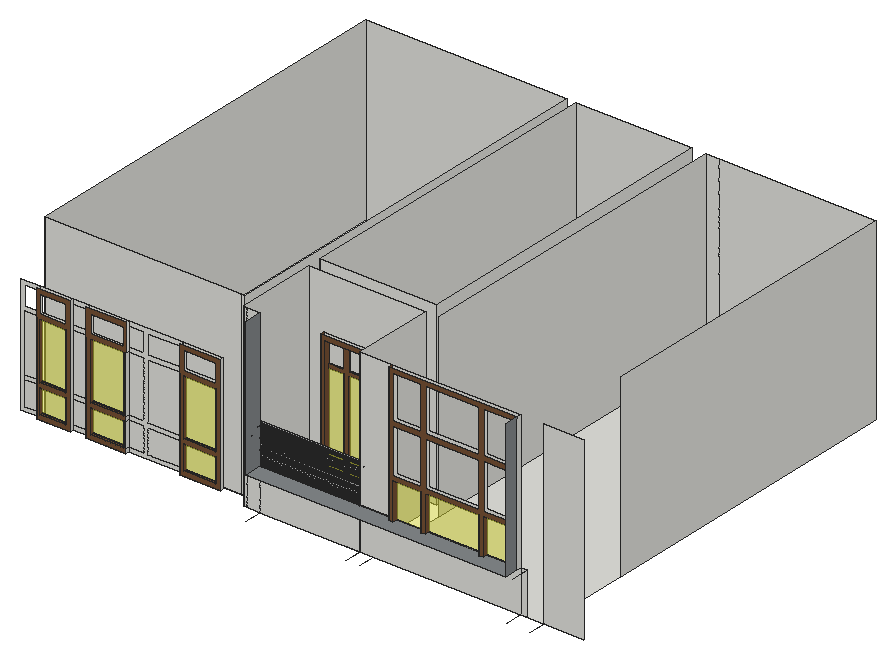
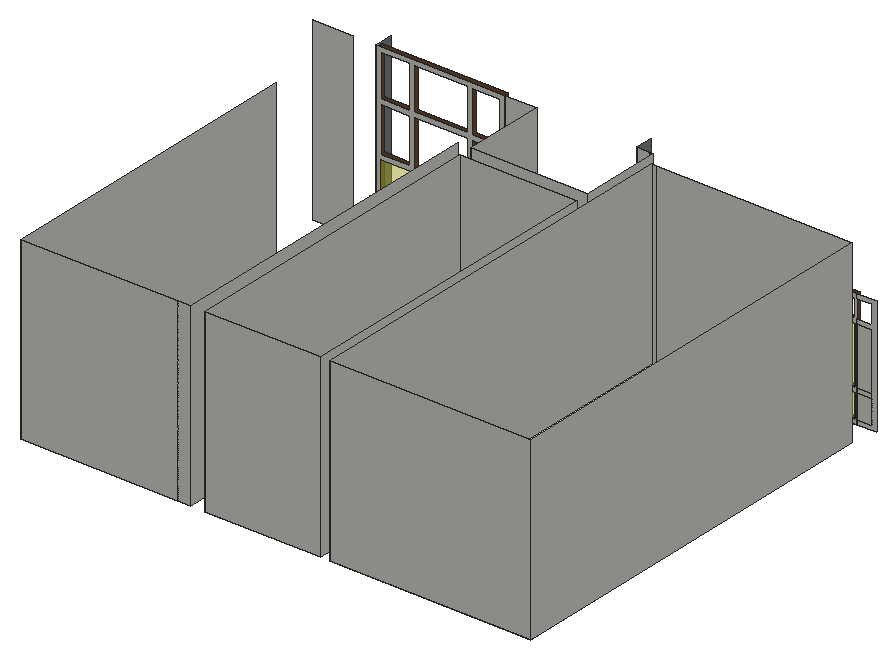
# SketchUp Ruby script. Lengths in inches.
U = 1.inch
M = Sketchup.active_model
def pt(a) = Geom::Point3d.new(a.map { |v| v * U })
def face(e, loops, mat)
  f = e.add_face(loops[0].map { |a| pt(a) })
  loops[1..].each { |l| e.add_face(l.map { |a| pt(a) }).erase! }
  f.material = f.back_material = mat if mat
  f
end
# faces: each face lists its corners as indices into pts; further lists are holes
def faces(e, pts, list, mat = nil) = list.each { |f| face(e, (f[0].is_a?(Array) ? f : [f]).map { |l| l.map { |i| pts[i] } }, mat) }
# xy, xz, yz: faces in a plane at the given z, y or x. An outline is a flat list of corners, or four numbers for a rectangle; further outlines are holes
def ring(l) = l.size == 4 ? [[l[0], l[1]], [l[2], l[1]], [l[2], l[3]], [l[0], l[3]]] : l.each_slice(2).to_a
def flat(e, list, mat, &to3) = list.each { |f| face(e, (f[0].is_a?(Array) ? f : [f]).map { |l| ring(l).map { |u, v| to3.(u, v) } }, mat) }
def xy(e, z, list, mat = nil) = flat(e, list, mat) { |x, y| [x, y, z] }
def xz(e, y, list, mat = nil) = flat(e, list, mat) { |x, z| [x, y, z] }
def yz(e, x, list, mat = nil) = flat(e, list, mat) { |y, z| [x, y, z] }
def lines(e, pts, list) = list.each { |a, b| e.add_line(pt(pts[a]), pt(pts[b])) }
# prism: a flat outline (further loops are holes) pulled along v
def prism(e, loops, v, mat = nil)
  f = face(e, loops, mat); d = Geom::Vector3d.new(v.map { |x| x * U })
  f.pushpull(f.normal.samedirection?(d) ? d.length : -d.length)
end
def box(e, o, s, mat = nil) = prism(e, [[o, [o[0] + s[0], o[1], o[2]], [o[0] + s[0], o[1] + s[1], o[2]], [o[0], o[1] + s[1], o[2]]]], [0, 0, s[2]], mat)
def at(x, y, z, deg = 0) = Geom::Transformation.translation(pt([x, y, z])) * Geom::Transformation.rotation(ORIGIN, Z_AXIS, deg.degrees)
def axes(o, x, y, z) = Geom::Transformation.new([*x, 0, *y, 0, *z, 0, *pt(o).to_a, 1])
def part(name) = M.definitions.add(name)
# library, detail: a bought-in or finely detailed component or shape, given as its bounding box
def library(name, o, s) = part(name).tap { |d| box(d.entities, o, s) }
def detail(e, o, s) = box(e.add_group.entities, o, s)
def put(e, d, t, mat = nil) = e.add_instance(d, t).tap { |i| i.material = mat if mat }
def group(e, t, mat = nil) = e.add_group.tap { |g| g.transformation = t; g.material = mat if mat }.entities
root = M.entities
M.materials.add("[0132_LightGray]").color = [169, 169, 169]
M.materials.add("[Blacktop Old 01]").color = [132, 136, 139]
M.materials.add("[Sandstone]").color = [118, 81, 52]
M.materials.add("[Translucent Glass Blue]").color = [254, 255, 58]
M.materials["[Translucent Glass Blue]"].alpha = 0.5
xy(root,123,[[149.5625,107.5,227.6875,116.5],[236.6875,107.5,351,385.8125],[9,116.5,143.5625,385.8125],[149.5625,116.5,227.6875,116.5,227.6875,162.625,219.46,162.625,219.46,159.625,216.46,159.625,216.46,162.625,208.9,162.625,208.9,161.625,205.9,161.625,205.9,162.625,198.65,162.625,198.65,161.625,195.65,161.625,195.65,162.625,176.59,162.625,176.59,161.625,173.59,161.625,173.59,162.625,162.46,162.625,162.46,159.625,159.46,159.625,159.46,162.625,149.5625,162.625],[173.59,161.625,176.59,162.625],
  [195.65,161.625,198.65,162.625],[205.9,161.625,208.9,162.625],[149.5625,171.625,227.6875,385.8125]])
xy(root,128.33,[[108.79,105.5,135.89,107.5]])
xy(root,128.33,[[12.9375,105.5,35.3125,107.5],[45.625,105.5,72.45,107.5]],"[Sandstone]")
xy(root,131.33,[[14.63,105.5,32.375,107.5],[48.83,105.5,70.95,107.5],[111.24,105.5,132.89,107.5]],"[Sandstone]")
xy(root,147.46,[[14.63,105.5,32.375,107.5],[48.83,105.5,70.95,107.5],[111.24,105.5,132.89,107.5]],"[Sandstone]")
xy(root,150.46,[[14.63,105.5,32.375,107.5],[48.83,105.5,70.95,107.5],[111.24,105.5,132.89,107.5]],"[Sandstone]")
xy(root,150.99,[[249.13,104.5,252.13,107.5],[270.95,104.5,273.95,107.5],[309.9,104.5,312.9,107.5],[332.27,104.5,335.27,107.5]])
xy(root,150.99,[[160.6875,95.5,335.27,95.5,335.27,104.5,332.27,104.5,332.27,107.5,312.9,107.5,312.9,104.5,309.9,104.5,309.9,107.5,273.95,107.5,273.95,104.5,270.95,104.5,270.95,107.5,252.13,107.5,252.13,104.5,249.13,104.5,249.13,107.5,160.6875,107.5]],"[Blacktop Old 01]")
xz(root,104.5,[[[249.13,150.99,252.13,150.99,252.13,175.36,270.95,175.36,270.95,150.99,273.95,150.99,273.95,175.36,309.9,175.36,309.9,150.99,312.9,150.99,312.9,175.36,332.27,175.36,332.27,150.99,335.27,150.99,335.27,243,249.13,243],[273.95,178.36,309.9,208.5625],[273.95,211.5625,309.9,240],[312.9,178.36,332.27,208.5625],[252.13,178.36,270.95,208.5625],[312.9,211.5625,332.27,240],[252.13,211.5625,270.95,240]]],"[Sandstone]")
xz(root,105.5,[[[12.9375,128.33,35.3125,207.1],[14.63,150.46,32.375,188.6],[14.63,131.33,32.375,147.46],[14.63,191.6,32.375,204.1]],[[45.625,128.33,72.45,207.1],[48.83,150.46,70.95,188.6],[48.83,131.33,70.95,147.46],[48.83,191.6,70.95,204.1]],[[108.79,128.33,135.89,207.1],[111.24,150.46,132.89,188.6],[111.24,131.33,132.89,147.46],[111.24,191.6,132.89,204.1]]],"[Sandstone]")
xz(root,107.5,[[149.5625,123,151.6875,243],[151.6875,123,160.6875,243],[160.6875,123,227.6875,150.99],[227.6875,123,335.27,150.99],[335.27,123,339.25,150.99],
  [351,123,377.5,243],[0,128.33,0,207.1,12.9375,207.1,12.9375,204.1,3,204.1,3,191.6,12.9375,191.6,12.9375,188.6,3,188.6,3,131.33,12.9375,131.33,12.9375,128.33],[[12.9375,128.33,35.3125,207.1],[14.63,150.46,32.375,188.6],[14.63,131.33,32.375,147.46],[14.63,191.6,32.375,204.1]],[35.3125,128.33,35.3125,207.1,45.625,207.1,45.625,204.1,35.375,204.1,35.375,191.6,45.625,191.6,45.625,188.6,35.375,188.6,35.375,150.46,45.625,150.46,45.625,147.46,35.375,147.46,35.375,131.33,45.625,131.33,45.625,128.33],[[45.625,128.33,72.45,207.1],[48.83,150.46,70.95,188.6],[48.83,131.33,70.95,147.46],[48.83,191.6,70.95,204.1]],
  [72.45,128.33,72.45,131.33,82.75,131.33,82.75,147.46,72.45,147.46,72.45,150.46,82.75,150.46,82.75,188.6,72.45,188.6,72.45,191.6,82.75,191.6,82.75,204.1,72.45,204.1,72.45,207.1,108.79,207.1,108.79,204.1,85.75,204.1,85.75,191.6,108.79,191.6,108.79,188.6,85.75,188.6,85.75,150.46,108.79,150.46,108.79,147.46,85.75,147.46,85.75,131.33,108.79,131.33,108.79,128.33],[[108.79,128.33,135.89,207.1],[111.24,150.46,132.89,188.6],[111.24,131.33,132.89,147.46],[111.24,191.6,132.89,204.1]],[3,131.33,12.9375,147.46],[35.375,131.33,45.625,147.46],[72.45,131.33,82.75,147.46],
  [85.75,131.33,108.79,147.46],[3,147.46,12.9375,150.46],[3,150.46,12.9375,188.6],[35.375,150.46,45.625,188.6],[72.45,150.46,82.75,188.6],
  [85.75,150.46,108.79,188.6],[227.6875,150.99,249.13,243],[[249.13,150.99,249.13,243,335.27,243,335.27,150.99,332.27,150.99,332.27,175.36,312.9,175.36,312.9,150.99,309.9,150.99,309.9,175.36,273.95,175.36,273.95,150.99,270.95,150.99,270.95,175.36,252.13,175.36,252.13,150.99],[273.95,178.36,309.9,208.5625],[273.95,211.5625,309.9,240],[312.9,178.36,332.27,208.5625],[252.13,178.36,270.95,208.5625],[312.9,211.5625,332.27,240],[252.13,211.5625,270.95,240]]])
xz(root,107.5,[[14.63,131.33,32.375,147.46],[48.83,131.33,70.95,147.46],[111.24,131.33,132.89,147.46],[14.63,150.46,32.375,188.6],[48.83,150.46,70.95,188.6],
  [111.24,150.46,132.89,188.6],[252.13,150.99,270.95,175.36],[273.95,150.99,309.9,175.36],[312.9,150.99,332.27,175.36]],"[Translucent Glass Blue]")
xz(root,116.5,[[9,123,140.5625,243],[140.5625,123,143.5625,243]])
xz(root,159.625,[[159.46,123,162.46,123,162.46,204,216.46,204,216.46,123,219.46,123,219.46,207,159.46,207]],"[Sandstone]")
xz(root,161.625,[[173.59,123,176.59,123,176.59,186.83,195.65,186.83,195.65,123,198.65,123,198.65,186.83,205.9,186.83,205.9,123,208.9,123,208.9,186.83,216.46,186.83,216.46,189.41,208.9,189.41,208.9,204,205.9,204,205.9,189.41,198.65,189.41,198.65,204,195.65,204,195.65,189.41,176.59,189.41,176.59,204,173.59,204,173.59,189.41,162.46,189.41,162.46,186.83,173.59,186.83]],"[Sandstone]")
xz(root,162.625,[[149.5625,123,159.46,123,159.46,207,219.46,207,219.46,123,227.6875,123,227.6875,243,149.5625,243],[173.59,123,173.59,186.83,162.46,186.83,162.46,189.41,173.59,189.41,173.59,204,176.59,204,176.59,189.41,195.65,189.41,195.65,204,198.65,204,198.65,189.41,205.9,189.41,205.9,204,208.9,204,208.9,189.41,216.46,189.41,216.46,186.83,208.9,186.83,208.9,123,205.9,123,205.9,186.83,198.65,186.83,198.65,123,195.65,123,195.65,186.83,176.59,186.83,176.59,123]])
xz(root,162.625,[[162.46,123,173.59,186.83],[176.59,123,195.65,186.83],[198.65,123,205.9,186.83],[208.9,123,216.46,186.83]],"[Translucent Glass Blue]")
xz(root,171.625,[[149.5625,123,227.6875,243]])
xz(root,385.8125,[[9,123,143.5625,243],[149.5625,123,227.6875,243],[236.6875,123,245.6875,243],[245.6875,123,351,243]])
yz(root,9,[[116.5,123,385.8125,243]])
yz(root,12.9375,[[105.5,128.33,107.5,131.33],[105.5,131.33,107.5,147.46],[105.5,147.46,107.5,150.46],[105.5,150.46,107.5,188.6]])
yz(root,14.63,[[105.5,131.33,107.5,147.46],[105.5,150.46,107.5,188.6]],"[Sandstone]")
yz(root,32.375,[[105.5,131.33,107.5,147.46],[105.5,150.46,107.5,188.6]],"[Sandstone]")
yz(root,35.3125,[[105.5,128.33,107.5,207.1]])
yz(root,45.625,[[105.5,128.33,107.5,131.33],[105.5,131.33,107.5,147.46],[105.5,147.46,107.5,150.46],[105.5,150.46,107.5,188.6]])
yz(root,48.83,[[105.5,131.33,107.5,147.46],[105.5,150.46,107.5,188.6]],"[Sandstone]")
yz(root,70.95,[[105.5,131.33,107.5,147.46],[105.5,150.46,107.5,188.6]],"[Sandstone]")
yz(root,72.45,[[105.5,128.33,107.5,131.33],[105.5,131.33,107.5,147.46],[105.5,147.46,107.5,150.46],[105.5,150.46,107.5,188.6]])
yz(root,108.79,[[105.5,128.33,107.5,131.33],[105.5,131.33,107.5,147.46],[105.5,147.46,107.5,150.46],[105.5,150.46,107.5,188.6]])
yz(root,111.24,[[105.5,131.33,107.5,147.46],[105.5,150.46,107.5,188.6]],"[Sandstone]")
yz(root,132.89,[[105.5,131.33,107.5,147.46],[105.5,150.46,107.5,188.6]],"[Sandstone]")
yz(root,135.89,[[105.5,128.33,107.5,207.1]])
yz(root,143.5625,[[116.5,123,385.8125,243]])
yz(root,149.5625,[[[107.5,123,162.625,243],[111.46,136.84,110.83,136.92,110.24,137.16,109.74,137.55,109.35,138.06,109.11,138.64,109.02,139.27,109.11,139.91,109.35,140.49,109.74,141,110.24,141.39,110.83,141.63,111.46,141.71,112.09,141.63,112.68,141.39,113.18,141,113.57,140.49,113.8125,139.91,113.9,139.27,113.8125,138.64,113.57,138.06,113.18,137.55,112.68,137.16,112.09,136.92],[111.46,143.96,110.83,144.04,110.24,144.29,109.74,144.68,109.35,145.18,109.11,145.77,109.02,146.4,109.11,147.03,109.35,147.62,109.74,148.12,110.24,148.51,110.83,148.75,111.46,148.84,112.09,148.75,112.68,148.51,113.18,148.12,113.57,147.62,113.8125,147.03,113.9,146.4,113.8125,145.77,113.57,145.18,113.18,144.68,112.68,144.29,112.09,144.04],[111.46,151.09,110.83,151.17,110.24,151.41,109.74,151.8,109.35,152.31,109.11,152.89,109.02,153.52,109.11,154.16,109.35,154.74,109.74,155.25,110.24,155.64,110.83,155.88,111.46,155.96,112.09,155.88,112.68,155.64,113.18,155.25,113.57,154.74,113.8125,154.16,113.9,153.52,113.8125,152.89,113.57,152.31,113.18,151.8,112.68,151.41,112.09,151.17],[111.46,158.21,110.83,158.29,110.24,158.54,109.74,158.93,109.35,159.43,109.11,160.02,109.02,160.65,109.11,161.28,109.35,161.87,109.74,162.37,110.24,162.76,110.83,163,111.46,163.09,112.09,163,112.68,162.76,113.18,162.37,113.57,161.87,113.8125,161.28,113.9,160.65,113.8125,160.02,113.57,159.43,113.18,158.93,112.68,158.54,112.09,158.29],[111.46,165.34,110.83,165.42,110.24,165.66,109.74,166.05,109.35,166.56,109.11,167.14,109.02,167.77,109.11,168.41,109.35,168.99,109.74,169.5,110.24,169.89,110.83,170.13,111.46,170.21,112.09,170.13,112.68,169.89,113.18,169.5,113.57,168.99,113.8125,168.41,113.9,167.77,113.8125,167.14,113.57,166.56,113.18,166.05,112.68,165.66,112.09,165.42],[111.46,172.46,110.83,172.54,110.24,172.79,109.74,173.18,109.35,173.68,109.11,174.27,109.02,174.9,109.11,175.53,109.35,176.12,109.74,176.62,110.24,177.01,110.83,177.25,111.46,177.34,112.09,177.25,112.68,177.01,113.18,176.62,113.57,176.12,113.8125,175.53,113.9,174.9,113.8125,174.27,113.57,173.68,113.18,173.18,112.68,172.79,112.09,172.54]],[171.625,123,385.8125,243],[111.46,136.84,112.09,136.92,112.68,137.16,113.18,137.55,113.57,138.06,113.8125,138.64,113.9,139.27,113.8125,139.91,113.57,140.49,113.18,141,112.68,141.39,112.09,141.63,111.46,141.71,110.83,141.63,110.24,141.39,109.74,141,109.35,140.49,109.11,139.91,109.02,139.27,109.11,138.64,109.35,138.06,109.74,137.55,110.24,137.16,110.83,136.92]])
yz(root,159.46,[[159.625,123,162.625,207]],"[Sandstone]")
yz(root,160.6875,[[95.5,150.99,107.5,243]],"[Blacktop Old 01]")
yz(root,162.46,[[159.625,123,162.625,123,162.625,186.83,161.625,186.83,161.625,189.41,162.625,189.41,162.625,204,159.625,204]],"[Sandstone]")
yz(root,173.59,[[161.625,123,162.625,186.83]],"[Sandstone]")
yz(root,176.59,[[161.625,123,162.625,186.83]],"[Sandstone]")
yz(root,195.65,[[161.625,123,162.625,186.83]],"[Sandstone]")
yz(root,198.65,[[161.625,123,162.625,186.83]],"[Sandstone]")
yz(root,205.9,[[161.625,123,162.625,186.83]],"[Sandstone]")
yz(root,208.9,[[161.625,123,162.625,186.83]],"[Sandstone]")
yz(root,216.46,[[159.625,123,159.625,204,162.625,204,162.625,189.41,161.625,189.41,161.625,186.83,162.625,186.83,162.625,123]],"[Sandstone]")
yz(root,219.46,[[159.625,123,162.625,207]],"[Sandstone]")
yz(root,227.6875,[[[107.5,123,162.625,243],[111.46,165.34,112.09,165.42,112.68,165.66,113.18,166.05,113.57,166.56,113.8125,167.14,113.9,167.77,113.8125,168.41,113.57,168.99,113.18,169.5,112.68,169.89,112.09,170.13,111.46,170.21,110.83,170.13,110.24,169.89,109.74,169.5,109.35,168.99,109.11,168.41,109.02,167.77,109.11,167.14,109.35,166.56,109.74,166.05,110.24,165.66,110.83,165.42],[111.46,143.96,112.09,144.04,112.68,144.29,113.18,144.68,113.57,145.18,113.8125,145.77,113.9,146.4,113.8125,147.03,113.57,147.62,113.18,148.12,112.68,148.51,112.09,148.75,111.46,148.84,110.83,148.75,110.24,148.51,109.74,148.12,109.35,147.62,109.11,147.03,109.02,146.4,109.11,145.77,109.35,145.18,109.74,144.68,110.24,144.29,110.83,144.04]],[171.625,123,385.8125,243]])
yz(root,229.5625,[[111.46,151.09,112.09,151.17,112.68,151.41,113.18,151.8,113.57,152.31,113.8125,152.89,113.9,153.52,113.8125,154.16,113.57,154.74,113.18,155.25,112.68,155.64,112.09,155.88,111.46,155.96,110.83,155.88,110.24,155.64,109.74,155.25,109.35,154.74,109.11,154.16,109.02,153.52,109.11,152.89,109.35,152.31,109.74,151.8,110.24,151.41,110.83,151.17]])
yz(root,232,[[111.46,158.21,112.09,158.29,112.68,158.54,113.18,158.93,113.57,159.43,113.8125,160.02,113.9,160.65,113.8125,161.28,113.57,161.87,113.18,162.37,112.68,162.76,112.09,163,111.46,163.09,110.83,163,110.24,162.76,109.74,162.37,109.35,161.87,109.11,161.28,109.02,160.65,109.11,160.02,109.35,159.43,109.74,158.93,110.24,158.54,110.83,158.29]])
yz(root,234.5625,[[111.46,172.46,112.09,172.54,112.68,172.79,113.18,173.18,113.57,173.68,113.8125,174.27,113.9,174.9,113.8125,175.53,113.57,176.12,113.18,176.62,112.68,177.01,112.09,177.25,111.46,177.34,110.83,177.25,110.24,177.01,109.74,176.62,109.35,176.12,109.11,175.53,109.02,174.9,109.11,174.27,109.35,173.68,109.74,173.18,110.24,172.79,110.83,172.54]])
yz(root,236.6875,[[162.625,123,385.8125,243]])
yz(root,249.13,[[104.5,150.99,107.5,243]],"[Sandstone]")
yz(root,252.13,[[104.5,150.99,107.5,175.36]],"[Sandstone]")
yz(root,270.95,[[104.5,150.99,107.5,175.36]],"[Sandstone]")
yz(root,273.95,[[104.5,150.99,107.5,175.36]],"[Sandstone]")
yz(root,309.9,[[104.5,150.99,107.5,175.36]],"[Sandstone]")
yz(root,312.9,[[104.5,150.99,107.5,175.36]],"[Sandstone]")
yz(root,332.27,[[104.5,150.99,107.5,175.36]],"[Sandstone]")
yz(root,335.27,[[104.5,150.99,107.5,243]])
yz(root,335.27,[[95.5,150.99,104.5,243]],"[Blacktop Old 01]")
yz(root,351,[[171.625,123,385.8125,243]])
p = [[149.5625,110.24,144.29],[149.5625,110.83,144.04],[227.6875,110.83,144.04],[227.6875,110.24,144.29],[149.5625,111.46,143.96],[227.6875,111.46,143.96],
  [149.5625,112.09,144.04],[227.6875,112.09,144.04],[149.5625,112.68,144.29],[227.6875,112.68,144.29],[149.5625,109.74,144.68],[227.6875,109.74,144.68],
  [149.5625,113.18,144.68],[227.6875,113.18,144.68],[149.5625,109.35,145.18],[227.6875,109.35,145.18],[149.5625,113.57,145.18],[227.6875,113.57,145.18],
  [149.5625,109.11,145.77],[227.6875,109.11,145.77],[149.5625,113.8125,145.77],[227.6875,113.8125,145.77],[149.5625,109.02,146.4],[227.6875,109.02,146.4],
  [149.5625,113.9,146.4],[227.6875,113.9,146.4],[149.5625,109.11,147.03],[227.6875,109.11,147.03],[149.5625,113.8125,147.03],[227.6875,113.8125,147.03],
  [149.5625,109.35,147.62],[227.6875,109.35,147.62],[149.5625,113.57,147.62],[227.6875,113.57,147.62],[149.5625,109.74,148.12],[227.6875,109.74,148.12],
  [149.5625,113.18,148.12],[227.6875,113.18,148.12],[149.5625,110.24,148.51],[227.6875,110.24,148.51],[149.5625,112.68,148.51],[227.6875,112.68,148.51],
  [149.5625,110.83,148.75],[227.6875,110.83,148.75],[149.5625,112.09,148.75],[227.6875,112.09,148.75],[149.5625,111.46,148.84],[227.6875,111.46,148.84],
  [149.5625,110.83,151.17],[149.5625,111.46,151.09],[229.5625,111.46,151.09],[229.5625,110.83,151.17],[149.5625,112.09,151.17],[229.5625,112.09,151.17],
  [149.5625,110.24,151.41],[229.5625,110.24,151.41],[149.5625,112.68,151.41],[229.5625,112.68,151.41],[149.5625,109.74,151.8],[229.5625,109.74,151.8],
  [149.5625,113.18,151.8],[229.5625,113.18,151.8],[149.5625,109.35,152.31],[229.5625,109.35,152.31],[149.5625,113.57,152.31],[229.5625,113.57,152.31],
  [149.5625,109.11,152.89],[229.5625,109.11,152.89],[149.5625,113.8125,152.89],[229.5625,113.8125,152.89],[149.5625,109.02,153.52],[229.5625,109.02,153.52],
  [149.5625,113.9,153.52],[229.5625,113.9,153.52],[149.5625,109.11,154.16],[229.5625,109.11,154.16],[149.5625,113.8125,154.16],[229.5625,113.8125,154.16],
  [149.5625,109.35,154.74],[229.5625,109.35,154.74],[149.5625,113.57,154.74],[229.5625,113.57,154.74],[149.5625,109.74,155.25],[229.5625,109.74,155.25],
  [149.5625,113.18,155.25],[229.5625,113.18,155.25],[149.5625,110.24,155.64],[229.5625,110.24,155.64],[149.5625,112.68,155.64],[229.5625,112.68,155.64],
  [149.5625,110.83,155.88],[229.5625,110.83,155.88],[149.5625,112.09,155.88],[229.5625,112.09,155.88],[149.5625,111.46,155.96],[229.5625,111.46,155.96],
  [149.5625,110.83,158.29],[149.5625,111.46,158.21],[232,111.46,158.21],[232,110.83,158.29],[149.5625,112.09,158.29],[232,112.09,158.29],
  [149.5625,110.24,158.54],[232,110.24,158.54],[149.5625,112.68,158.54],[232,112.68,158.54],[149.5625,109.74,158.93],[232,109.74,158.93],
  [149.5625,113.18,158.93],[232,113.18,158.93],[149.5625,109.35,159.43],[232,109.35,159.43],[149.5625,113.57,159.43],[232,113.57,159.43],
  [149.5625,109.11,160.02],[232,109.11,160.02],[149.5625,113.8125,160.02],[232,113.8125,160.02],[149.5625,109.02,160.65],[232,109.02,160.65],
  [149.5625,113.9,160.65],[232,113.9,160.65],[149.5625,109.11,161.28],[232,109.11,161.28],[149.5625,113.8125,161.28],[232,113.8125,161.28],
  [149.5625,109.35,161.87],[232,109.35,161.87],[149.5625,113.57,161.87],[232,113.57,161.87],[149.5625,109.74,162.37],[232,109.74,162.37],
  [149.5625,113.18,162.37],[232,113.18,162.37],[149.5625,110.24,162.76],[232,110.24,162.76],[149.5625,112.68,162.76],[232,112.68,162.76],
  [149.5625,110.83,163],[232,110.83,163],[149.5625,112.09,163],[232,112.09,163],[149.5625,111.46,163.09],[232,111.46,163.09],
  [149.5625,110.83,165.42],[149.5625,111.46,165.34],[227.6875,111.46,165.34],[227.6875,110.83,165.42],[149.5625,112.09,165.42],[227.6875,112.09,165.42],
  [149.5625,110.24,165.66],[227.6875,110.24,165.66],[149.5625,112.68,165.66],[227.6875,112.68,165.66],[149.5625,109.74,166.05],[227.6875,109.74,166.05],
  [149.5625,113.18,166.05],[227.6875,113.18,166.05],[149.5625,109.35,166.56],[227.6875,109.35,166.56],[149.5625,113.57,166.56],[227.6875,113.57,166.56],
  [149.5625,109.11,167.14],[227.6875,109.11,167.14],[149.5625,113.8125,167.14],[227.6875,113.8125,167.14],[149.5625,109.02,167.77],[227.6875,109.02,167.77],
  [149.5625,113.9,167.77],[227.6875,113.9,167.77],[149.5625,109.11,168.41],[227.6875,109.11,168.41],[149.5625,113.8125,168.41],[227.6875,113.8125,168.41],
  [149.5625,109.35,168.99],[227.6875,109.35,168.99],[149.5625,113.57,168.99],[227.6875,113.57,168.99],[149.5625,109.74,169.5],[227.6875,109.74,169.5],
  [149.5625,113.18,169.5],[227.6875,113.18,169.5],[149.5625,110.24,169.89],[227.6875,110.24,169.89],[149.5625,112.68,169.89],[227.6875,112.68,169.89],
  [149.5625,110.83,170.13],[227.6875,110.83,170.13],[149.5625,112.09,170.13],[227.6875,112.09,170.13],[149.5625,111.46,170.21],[227.6875,111.46,170.21],
  [149.5625,110.24,172.79],[149.5625,110.83,172.54],[234.5625,110.83,172.54],[234.5625,110.24,172.79],[149.5625,111.46,172.46],[234.5625,111.46,172.46],
  [149.5625,112.09,172.54],[234.5625,112.09,172.54],[149.5625,112.68,172.79],[234.5625,112.68,172.79],[149.5625,109.74,173.18],[234.5625,109.74,173.18],
  [149.5625,113.18,173.18],[234.5625,113.18,173.18],[149.5625,109.35,173.68],[234.5625,109.35,173.68],[149.5625,113.57,173.68],[234.5625,113.57,173.68],
  [339.25,95.5,150.99],[339.25,107.5,150.99],[236.6875,107.5,123],[236.6875,95.5,123],[227.6875,107.5,123],[227.6875,95.5,123],
  [160.6875,107.5,123],[160.6875,95.5,123],[351,107.5,123],[351,95.5,123],[335.27,107.5,123],[335.27,95.5,123]]
faces(root,p,[[0,1,2,3],[1,4,5,2],[4,6,7,5],[6,8,9,7],[10,0,3,11],[8,12,13,9],[14,10,11,15],[12,16,17,13],
  [18,14,15,19],[16,20,21,17],[22,18,19,23],[20,24,25,21],[26,22,23,27],[24,28,29,25],[30,26,27,31],[28,32,33,29],
  [34,30,31,35],[32,36,37,33],[38,34,35,39],[36,40,41,37],[42,38,39,43],[40,44,45,41],[46,42,43,47],[44,46,47,45],
  [48,49,50,51],[49,52,53,50],[54,48,51,55],[52,56,57,53],[58,54,55,59],[56,60,61,57],[62,58,59,63],[60,64,65,61],
  [66,62,63,67],[64,68,69,65],[70,66,67,71],[68,72,73,69],[74,70,71,75],[72,76,77,73],[78,74,75,79],[76,80,81,77],
  [82,78,79,83],[80,84,85,81],[86,82,83,87],[84,88,89,85],[90,86,87,91],[88,92,93,89],[94,90,91,95],[92,94,95,93],
  [96,97,98,99],[97,100,101,98],[102,96,99,103],[100,104,105,101],[106,102,103,107],[104,108,109,105],[110,106,107,111],[108,112,113,109],
  [114,110,111,115],[112,116,117,113],[118,114,115,119],[116,120,121,117],[122,118,119,123],[120,124,125,121],[126,122,123,127],[124,128,129,125],
  [130,126,127,131],[128,132,133,129],[134,130,131,135],[132,136,137,133],[138,134,135,139],[136,140,141,137],[142,138,139,143],[140,142,143,141],
  [144,145,146,147],[145,148,149,146],[150,144,147,151],[148,152,153,149],[154,150,151,155],[152,156,157,153],[158,154,155,159],[156,160,161,157],
  [162,158,159,163],[160,164,165,161],[166,162,163,167],[164,168,169,165],[170,166,167,171],[168,172,173,169],[174,170,171,175],[172,176,177,173],
  [178,174,175,179],[176,180,181,177],[182,178,179,183],[180,184,185,181],[186,182,183,187],[184,188,189,185],[190,186,187,191],[188,190,191,189],
  [192,193,194,195],[193,196,197,194],[196,198,199,197],[198,200,201,199],[202,192,195,203],[200,204,205,201],[206,202,203,207],[204,208,209,205]],"[0132_LightGray]")
lines(root,p,[[210,211],[212,213],[214,215],[216,217],[218,219],[220,221]])
